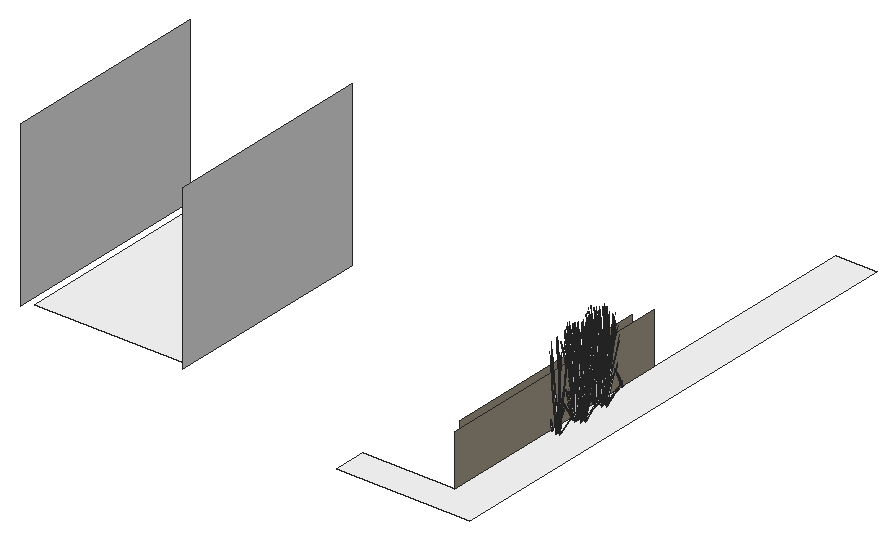
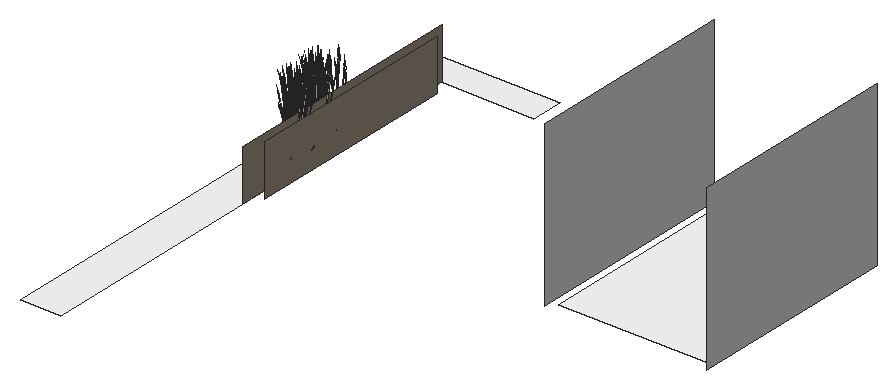
# SketchUp Ruby script. Lengths in inches.
U = 1.inch
M = Sketchup.active_model
def pt(a) = Geom::Point3d.new(a.map { |v| v * U })
def face(e, loops, mat)
  f = e.add_face(loops[0].map { |a| pt(a) })
  loops[1..].each { |l| e.add_face(l.map { |a| pt(a) }).erase! }
  f.material = f.back_material = mat if mat
  f
end
# faces: each face lists its corners as indices into pts; further lists are holes
def faces(e, pts, list, mat = nil) = list.each { |f| face(e, (f[0].is_a?(Array) ? f : [f]).map { |l| l.map { |i| pts[i] } }, mat) }
# xy, xz, yz: faces in a plane at the given z, y or x. An outline is a flat list of corners, or four numbers for a rectangle; further outlines are holes
def ring(l) = l.size == 4 ? [[l[0], l[1]], [l[2], l[1]], [l[2], l[3]], [l[0], l[3]]] : l.each_slice(2).to_a
def flat(e, list, mat, &to3) = list.each { |f| face(e, (f[0].is_a?(Array) ? f : [f]).map { |l| ring(l).map { |u, v| to3.(u, v) } }, mat) }
def xy(e, z, list, mat = nil) = flat(e, list, mat) { |x, y| [x, y, z] }
def xz(e, y, list, mat = nil) = flat(e, list, mat) { |x, z| [x, y, z] }
def yz(e, x, list, mat = nil) = flat(e, list, mat) { |y, z| [x, y, z] }
def lines(e, pts, list) = list.each { |a, b| e.add_line(pt(pts[a]), pt(pts[b])) }
# prism: a flat outline (further loops are holes) pulled along v
def prism(e, loops, v, mat = nil)
  f = face(e, loops, mat); d = Geom::Vector3d.new(v.map { |x| x * U })
  f.pushpull(f.normal.samedirection?(d) ? d.length : -d.length)
end
def box(e, o, s, mat = nil) = prism(e, [[o, [o[0] + s[0], o[1], o[2]], [o[0] + s[0], o[1] + s[1], o[2]], [o[0], o[1] + s[1], o[2]]]], [0, 0, s[2]], mat)
def at(x, y, z, deg = 0) = Geom::Transformation.translation(pt([x, y, z])) * Geom::Transformation.rotation(ORIGIN, Z_AXIS, deg.degrees)
def axes(o, x, y, z) = Geom::Transformation.new([*x, 0, *y, 0, *z, 0, *pt(o).to_a, 1])
def part(name) = M.definitions.add(name)
# library, detail: a bought-in or finely detailed component or shape, given as its bounding box
def library(name, o, s) = part(name).tap { |d| box(d.entities, o, s) }
def detail(e, o, s) = box(e.add_group.entities, o, s)
def put(e, d, t, mat = nil) = e.add_instance(d, t).tap { |i| i.material = mat if mat }
def group(e, t, mat = nil) = e.add_group.tap { |g| g.transformation = t; g.material = mat if mat }.entities
root = M.entities
M.materials.add("LightPink_Translucent").color = [144, 107, 117]
M.materials["LightPink_Translucent"].alpha = 0.75
M.materials.add("M00_Soft_Cloud").color = [255, 255, 255]
M.materials.add("Plaster_04_1K").color = [142, 132, 117]
M.materials.add("[Metal_Corrogated_Shiny]").color = [193, 193, 193]
c1 = part("blade")
p = [[2.15,0.21,22],[0,0.17,0],[0.09,0.45,0],[2.18,0.31,22],[2.29,0.31,22],[0.38,0.45,0],
  [2.48,0.24,33],[2.49,0.24,33],[2.48,0.22,33]]
faces(c1.entities,p,[[0,1,2,3],[4,5,2,3],[6,3,4,7],[8,0,3,6]])
c2 = part("seeds")
p = [[0.3,-0.1,1.38],[-0.01,-0.03,1.59],[-0.01,-0.03,0.03],[0.14,-0.07,-0.07],[0.29,-0.03,3],[0.15,0.01,3.11]]
faces(c2.entities,p,[[0,1,2,3],[1,0,4,5]],"LightPink_Translucent")
c3 = part("blade with seeds")
put(c3.entities,c1,at(0,0,0))
put(c3.entities,c2,axes([2.4,0.25,30.99],[1.5799,-0.05474,1.17369],[-0.12525,1.92788,0.29478],[-0.07173,-0.02425,1.56792]))
xy(root,255,[[333.82,39.98,432,39.98,432,414.98,402,414.98,402,63.98,333.82,63.98],[78,82.09,186,225.98]],"M00_Soft_Cloud")
yz(root,72,[[75.98,255,231.98,375]],"[Metal_Corrogated_Shiny]")
yz(root,192,[[75.98,255,231.98,375]],"[Metal_Corrogated_Shiny]")
yz(root,396,[[75.98,255,234.98,292.64]],"Plaster_04_1K")
yz(root,402,[[63.98,255,246.98,292.64]],"Plaster_04_1K")
put(root,c3,axes([409.78,148.04,257.21],[-0.36864,0.55059,-0.44739],[-0.76598,-0.26498,0.21531],[0,0.12692,1.43643]))
put(root,c3,axes([408.89,148.84,257.06],[-0.51177,0.45928,-0.62353],[-0.63575,-0.41646,-0.16365],[-0.20507,0.11457,1.37633]))
put(root,c3,axes([409.8,149.62,257.33],[0.95122,0.19861,0.30756],[-0.23797,0.7099,-0.36492],[-0.15744,0.08885,1.64885]))
put(root,c3,axes([409.73,150.1,257.02],[-0.7111,0.30552,-0.49651],[-0.42504,-0.54784,0],[-0.16196,0.06958,1.57504]))
put(root,c3,axes([412.09,148.29,257.02],[0,0.61104,-0.49651],[-0.85008,0,0],[0,0.13917,1.57504]))
put(root,c3,axes([410.375,150,257.375],[0.47504,0.61229,0],[-0.79476,0.34146,-0.51607],[-0.18101,0.07777,1.63711]))
put(root,c3,axes([411.13,150.21,256.49],[0.05536,-0.08822,1.76342],[0.69692,-0.25981,-0.26939],[0.21129,0.13447,0.30037]))
put(root,c3,axes([410.21,148.2,257.09],[0.2786,0.55945,-0.69212],[-0.80253,0.20149,-0.18165],[0.03079,0.18945,1.52773]))
put(root,c3,axes([404.73,150.13,256.49],[0.10192,0.06105,1.76342],[0.17281,0.56562,-0.26939],[-0.22588,0.12062,0.30037]))
put(root,c3,axes([407.875,150.1875,256.49],[0.12297,-0.03325,1.76342],[0.73967,0.18301,-0.26939],[0.02163,0.20626,0.30037]))
put(root,c3,axes([408.77,166.76,256.49],[-0.12744,0.02202,1.76342],[-0.70477,-0.24781,-0.26939],[0.01183,-0.2067,0.30037]))
put(root,c3,axes([406.49,167.52,256.49],[-0.0736,0.08049,1.76342],[-0.74378,0.17355,-0.26939],[-0.17968,-0.15788,0.30037]))
put(root,c3,axes([407.72,169.73,257.1],[-0.31203,-0.62659,-0.69835],[0.89884,-0.22566,-0.18329],[-0.03449,-0.21218,1.54149]))
put(root,c3,axes([411.89,167.82,256.49],[-0.11372,-0.04814,1.76342],[-0.29211,-0.53779,-0.26939],[0.19706,-0.14594,0.30037]))
put(root,c3,axes([407.6,167.93,257.375],[-0.47504,-0.61229,0],[0.79476,-0.34146,-0.51607],[0.18101,-0.07777,1.63711]))
put(root,c3,axes([408.64,167.19,257.13],[-0.52505,0.35054,-0.03893],[-0.48109,-0.38392,-0.17649],[-0.03387,-0.10878,0.58215]))
put(root,c3,axes([405.88,169.64,257.02],[0,-0.61104,-0.49651],[0.85008,0,0],[0,-0.13917,1.57504]))
put(root,c3,axes([408.24,167.84,257.02],[0.7111,-0.30552,-0.49651],[0.42504,0.54784,0],[0.16196,-0.06958,1.57504]))
put(root,c3,axes([409.08,169.09,257.06],[0.51177,-0.45928,-0.62353],[0.63575,0.41646,-0.16365],[0.20507,-0.11457,1.37633]))
put(root,c3,axes([408.19,169.89,257.21],[0.36864,-0.55059,-0.44739],[0.76598,0.26498,0.21531],[0,-0.12692,1.43643]))
put(root,c3,axes([408.53,169.62,257.67],[-0.08854,-0.69723,-0.29095],[0.92215,-0.04216,-0.50002],[0.16238,-0.09287,1.59708]))
put(root,c3,axes([406.24,169.66,257.03],[0.53038,-0.38124,-0.30978],[0.53038,0.38124,0.30978],[0,-0.1228,1.38974]))
put(root,c3,axes([406.03,167.83,257.13],[-0.21918,0.49894,-0.03893],[-0.6746,-0.15348,-0.17649],[-0.10242,-0.08161,0.58215]))
put(root,c3,axes([408.1,170.35,257.67],[-0.85568,-0.29155,-0.29095],[0.41201,-0.61537,-0.50002],[-0.02689,-0.15109,1.59708]))
put(root,c3,axes([405.67,170.11,257.375],[-0.95008,0,0],[0,-0.68292,-0.51607],[0,-0.15554,1.63711]))
put(root,c3,axes([408.41,168.08,257.03],[0.70886,0.15119,-0.30978],[-0.17848,0.53243,0.30978],[0.1429,-0.0614,1.38974]))
put(root,c3,axes([406.4,169.93,257.33],[-0.70674,0.51372,0.30756],[-0.70717,-0.50832,-0.36492],[-0.02468,-0.14589,1.64885]))
put(root,c3,axes([408.32,171,257.4375],[0.20138,-0.72405,-0.23429],[0.95485,0.12621,0.51271],[-0.16685,-0.09999,1.5644]))
put(root,c3,axes([411.09,168.08,257.375],[0.47504,-0.61229,0],[0.79476,0.34146,-0.51607],[0.18101,0.07777,1.63711]))
put(root,c3,axes([408.25,170.7,257.21],[-0.45644,-0.51287,-0.44739],[0.69137,-0.36116,0.21531],[-0.14771,-0.06346,1.43643]))
put(root,c3,axes([408.35,169.98,257.36],[0.33034,0.68327,0.45755],[-0.94388,0.2376,0.17955],[0.01154,-0.12555,1.58856]))
put(root,c3,axes([412.96,170.5,256.98],[-0.48937,0.07333,1.41583],[-0.07789,-0.58369,0.08104],[0.34275,-0.08835,0.80566]))
put(root,c3,axes([413.86,169.99,257.26],[-0.47106,-0.39072,-0.06488],[0.51591,-0.35801,-0.29416],[0.14618,-0.02521,0.97024]))
put(root,c3,axes([409.53,170.04,257.21],[0,-0.70701,0],[0.95008,0,0],[0,0,1.79456]))
put(root,c3,axes([407.84,170.9,257.06],[-0.79037,-0.10018,-0.62353],[0.16679,-0.61794,-0.16365],[-0.23587,-0.07488,1.37633]))
put(root,c3,axes([409.08,169.59,257.36],[-0.62999,0.55453,0.45755],[-0.74845,-0.4895,0.17955],[0.15188,-0.05534,1.58856]))
put(root,c3,axes([409.77,170.59,257.3],[-0.70674,-0.52593,-0.06131],[0.70717,-0.52625,0],[-0.02468,-0.01837,1.75571]))
put(root,c3,axes([407.66,169.17,256.59],[-0.74787,0.24464,1.28929],[-0.23804,-0.70192,0.50096],[0.45924,0.01168,1.46642]))
put(root,c3,axes([408.43,170.65,257.36],[0.96033,0.12874,0.45755],[-0.19544,0.7271,0.17955],[-0.14034,-0.07021,1.58856]))
put(root,c3,axes([413.5,170.125,256.49],[-0.03971,-0.09277,1.76342],[0.27541,-0.54264,-0.26939],[0.27782,-0.00781,0.30037]))
put(root,c3,axes([405.3,170.03,256.49],[0.01927,0.0963,1.76342],[-0.38846,0.5029,-0.26939],[-0.27592,-0.02535,0.30037]))
put(root,c3,axes([407,171.84,257.03],[-0.17848,-0.53243,-0.30978],[0.70886,-0.15119,0.30978],[-0.1429,-0.0614,1.38974]))
put(root,c3,axes([409.59,169.53,257.67],[0.76714,-0.40567,-0.29095],[0.51013,0.57321,-0.50002],[0.18927,0.05821,1.59708]))
put(root,c3,axes([406.8,172.07,257.02],[-0.7111,-0.30552,-0.49651],[0.42504,-0.54784,0],[-0.16196,-0.06958,1.57504]))
put(root,c3,axes([411.53,168.45,257.02],[0.7111,0.30552,-0.49651],[-0.42504,0.54784,0],[0.16196,0.06958,1.57504]))
put(root,c3,axes([410.18,170.2,257.21],[0.85008,0,0],[0,0.63259,0],[0,0,1.78407]))
put(root,c3,axes([408.74,170.99,257.67],[-0.76714,0.40567,-0.29095],[-0.51013,-0.57321,-0.50002],[-0.18927,-0.05821,1.59708]))
put(root,c3,axes([411.33,168.68,257.03],[0.17848,0.53243,-0.30978],[-0.70886,0.15119,0.30978],[0.1429,0.0614,1.38974]))
put(root,c3,axes([409.14,171.67,257.2],[-0.24791,-0.5268,0],[0.70791,-0.18448,0],[0,0,1.54371]))
put(root,c3,axes([410.07,171.6,257.18],[0.79769,-0.20732,-0.19198],[0.2803,0.59721,0.00008],[0.08805,-0.02292,1.73897]))
put(root,c3,axes([410.16,170.47,257.21],[0.53038,0.39469,0],[-0.53038,0.39469,0],[0,0,1.69266]))
put(root,c3,axes([410.49,169.625,257.06],[0.79037,0.10018,-0.62353],[-0.16679,0.61794,-0.16365],[0.23587,0.07488,1.37633]))
put(root,c3,axes([408.96,171.91,257.2],[-0.76598,-0.27433,0],[0.36864,-0.57001,0],[0,0,1.62707]))
put(root,c3,axes([409.6,171.18,257.46],[-0.74193,-0.49181,-0.25192],[0.6243,-0.55226,0.5513],[-0.19979,0.05753,1.68216]))
put(root,c3,axes([410.01,170.32,257.29],[0,0.70667,-0.05637],[-0.95008,0,0],[0,0.02221,1.79368]))
put(root,c3,axes([410.08,169.82,257.21],[0.45644,0.51287,-0.44739],[-0.69137,0.36116,0.21531],[0.14771,0.06346,1.43643]))
put(root,c3,axes([407.24,172.44,257.375],[-0.47504,0.61229,0],[-0.79476,-0.34146,-0.51607],[-0.18101,-0.07777,1.63711]))
put(root,c3,axes([409.22,171.07,257.21],[-0.82508,0.03772,-0.44739],[-0.07462,-0.62614,0.21531],[-0.14771,0.06346,1.43643]))
put(root,c3,axes([409.83,171.92,257.2],[0.76598,0.27433,0],[-0.36864,0.57001,0],[0,0,1.74954]))
put(root,c3,axes([410.14,172.53,257.19],[-0.46912,-0.61443,-0.05142],[0.79476,-0.34146,0.51607],[-0.19584,0.0585,1.6363]))
put(root,c3,axes([409.56,171.6875,257.29],[0.33034,0.70197,-0.06012],[-0.94388,0.24598,0],[0.01154,0.02451,1.72173]))
put(root,c3,axes([409.92,172.45,257.03],[-0.70886,-0.15119,-0.30978],[0.17848,-0.53243,0.30978],[-0.1429,0.0614,1.38974]))
put(root,c3,axes([412.66,170.42,257.375],[0.95008,0,0],[0,0.68292,-0.51607],[0,0.15554,1.63711]))
put(root,c3,axes([412.29,170.77,257.2],[-0.94962,-0.00489,-0.04976],[0,-0.68292,0.49943],[-0.02984,0.15546,1.58352]))
put(root,c3,axes([410.23,170.17,257.67],[0.85568,0.29155,-0.29095],[-0.41201,0.61537,-0.50002],[0.02689,0.15109,1.59708]))
put(root,c3,axes([412.09,170.87,257.03],[-0.53038,0.38124,-0.30978],[-0.53038,-0.38124,0.30978],[0,0.1228,1.38974]))
put(root,c3,axes([409.8,170.9,257.67],[0.08854,0.69723,-0.29095],[-0.92215,0.04216,-0.50002],[-0.16238,0.09287,1.59708]))
put(root,c3,axes([410.14,170.63,257.21],[-0.36864,0.55059,-0.44739],[-0.76598,-0.26498,0.21531],[0,0.12692,1.43643]))
put(root,c3,axes([409.25,171.4375,257.06],[-0.51177,0.45928,-0.62353],[-0.63575,-0.41646,-0.16365],[-0.20507,0.11457,1.37633]))
put(root,c3,axes([410.16,172.21,257.33],[0.95122,0.19861,0.30756],[-0.23797,0.7099,-0.36492],[-0.15744,0.08885,1.64885]))
put(root,c3,axes([410.09,172.6875,257.02],[-0.7111,0.30552,-0.49651],[-0.42504,-0.54784,0],[-0.16196,0.06958,1.57504]))
put(root,c3,axes([412.45,170.88,257.02],[0,0.61104,-0.49651],[-0.85008,0,0],[0,0.13917,1.57504]))
put(root,c3,axes([410.74,172.59,257.375],[0.47504,0.61229,0],[-0.79476,0.34146,-0.51607],[-0.18101,0.07777,1.63711]))
put(root,c3,axes([411.49,172.8,256.49],[0.05536,-0.08822,1.76342],[0.69692,-0.25981,-0.26939],[0.21129,0.13447,0.30037]))
put(root,c3,axes([410.57,170.8,257.09],[0.2786,0.55945,-0.69212],[-0.80253,0.20149,-0.18165],[0.03079,0.18945,1.52773]))
put(root,c3,axes([405.09,172.73,256.49],[0.10192,0.06105,1.76342],[0.17281,0.56562,-0.26939],[-0.22588,0.12062,0.30037]))
put(root,c3,axes([408.24,172.78,256.49],[0.12297,-0.03325,1.76342],[0.73967,0.18301,-0.26939],[0.02163,0.20626,0.30037]))
put(root,c3,axes([406.75,188.89,256.49],[-0.12744,0.02202,1.76342],[-0.70477,-0.24781,-0.26939],[0.01183,-0.2067,0.30037]))
put(root,c3,axes([404.47,189.65,256.49],[-0.0736,0.08049,1.76342],[-0.74378,0.17355,-0.26939],[-0.17968,-0.15788,0.30037]))
put(root,c3,axes([405.7,191.86,257.1],[-0.31203,-0.62659,-0.69835],[0.89884,-0.22566,-0.18329],[-0.03449,-0.21218,1.54149]))
put(root,c3,axes([409.87,189.95,256.49],[-0.11372,-0.04814,1.76342],[-0.29211,-0.53779,-0.26939],[0.19706,-0.14594,0.30037]))
put(root,c3,axes([405.58,190.0625,257.375],[-0.47504,-0.61229,0],[0.79476,-0.34146,-0.51607],[0.18101,-0.07777,1.63711]))
put(root,c3,axes([406.62,189.32,257.13],[-0.52505,0.35054,-0.03893],[-0.48109,-0.38392,-0.17649],[-0.03387,-0.10878,0.58215]))
put(root,c3,axes([403.86,191.78,257.02],[0,-0.61104,-0.49651],[0.85008,0,0],[0,-0.13917,1.57504]))
put(root,c3,axes([406.22,189.97,257.02],[0.7111,-0.30552,-0.49651],[0.42504,0.54784,0],[0.16196,-0.06958,1.57504]))
put(root,c3,axes([407.07,191.22,257.06],[0.51177,-0.45928,-0.62353],[0.63575,0.41646,-0.16365],[0.20507,-0.11457,1.37633]))
put(root,c3,axes([406.17,192.02,257.21],[0.36864,-0.55059,-0.44739],[0.76598,0.26498,0.21531],[0,-0.12692,1.43643]))
put(root,c3,axes([406.51,191.75,257.67],[-0.08854,-0.69723,-0.29095],[0.92215,-0.04216,-0.50002],[0.16238,-0.09287,1.59708]))
put(root,c3,axes([404.23,191.79,257.03],[0.53038,-0.38124,-0.30978],[0.53038,0.38124,0.30978],[0,-0.1228,1.38974]))
put(root,c3,axes([404.01,189.96,257.13],[-0.21918,0.49894,-0.03893],[-0.6746,-0.15348,-0.17649],[-0.10242,-0.08161,0.58215]))
put(root,c3,axes([406.08,192.48,257.67],[-0.85568,-0.29155,-0.29095],[0.41201,-0.61537,-0.50002],[-0.02689,-0.15109,1.59708]))
put(root,c3,axes([403.65,192.24,257.375],[-0.95008,0,0],[0,-0.68292,-0.51607],[0,-0.15554,1.63711]))
put(root,c3,axes([406.39,190.21,257.03],[0.70886,0.15119,-0.30978],[-0.17848,0.53243,0.30978],[0.1429,-0.0614,1.38974]))
put(root,c3,axes([404.38,192.06,257.33],[-0.70674,0.51372,0.30756],[-0.70717,-0.50832,-0.36492],[-0.02468,-0.14589,1.64885]))
put(root,c3,axes([406.3,193.13,257.4375],[0.20138,-0.72405,-0.23429],[0.95485,0.12621,0.51271],[-0.16685,-0.09999,1.5644]))
put(root,c3,axes([409.08,190.22,257.375],[0.47504,-0.61229,0],[0.79476,0.34146,-0.51607],[0.18101,0.07777,1.63711]))
put(root,c3,axes([406.23,192.84,257.21],[-0.45644,-0.51287,-0.44739],[0.69137,-0.36116,0.21531],[-0.14771,-0.06346,1.43643]))
put(root,c3,axes([406.33,192.11,257.36],[0.33034,0.68327,0.45755],[-0.94388,0.2376,0.17955],[0.01154,-0.12555,1.58856]))
put(root,c3,axes([410.95,192.64,256.98],[-0.48937,0.07333,1.41583],[-0.07789,-0.58369,0.08104],[0.34275,-0.08835,0.80566]))
put(root,c3,axes([411.84,192.12,257.26],[-0.47106,-0.39072,-0.06488],[0.51591,-0.35801,-0.29416],[0.14618,-0.02521,0.97024]))
put(root,c3,axes([407.51,192.17,257.21],[0,-0.70701,0],[0.95008,0,0],[0,0,1.79456]))
put(root,c3,axes([405.82,193.03,257.06],[-0.79037,-0.10018,-0.62353],[0.16679,-0.61794,-0.16365],[-0.23587,-0.07488,1.37633]))
put(root,c3,axes([407.06,191.72,257.36],[-0.62999,0.55453,0.45755],[-0.74845,-0.4895,0.17955],[0.15188,-0.05534,1.58856]))
put(root,c3,axes([407.75,192.72,257.3],[-0.70674,-0.52593,-0.06131],[0.70717,-0.52625,0],[-0.02468,-0.01837,1.75571]))
put(root,c3,axes([405.64,191.3,256.59],[-0.74787,0.24464,1.28929],[-0.23804,-0.70192,0.50096],[0.45924,0.01168,1.46642]))
put(root,c3,axes([406.41,192.78,257.36],[0.96033,0.12874,0.45755],[-0.19544,0.7271,0.17955],[-0.14034,-0.07021,1.58856]))
put(root,c3,axes([411.48,192.25,256.49],[-0.03971,-0.09277,1.76342],[0.27541,-0.54264,-0.26939],[0.27782,-0.00781,0.30037]))
put(root,c3,axes([403.28,192.16,256.49],[0.01927,0.0963,1.76342],[-0.38846,0.5029,-0.26939],[-0.27592,-0.02535,0.30037]))
put(root,c3,axes([404.98,193.97,257.03],[-0.17848,-0.53243,-0.30978],[0.70886,-0.15119,0.30978],[-0.1429,-0.0614,1.38974]))
put(root,c3,axes([407.58,191.66,257.67],[0.76714,-0.40567,-0.29095],[0.51013,0.57321,-0.50002],[0.18927,0.05821,1.59708]))
put(root,c3,axes([404.79,194.2,257.02],[-0.7111,-0.30552,-0.49651],[0.42504,-0.54784,0],[-0.16196,-0.06958,1.57504]))
put(root,c3,axes([409.51,190.58,257.02],[0.7111,0.30552,-0.49651],[-0.42504,0.54784,0],[0.16196,0.06958,1.57504]))
put(root,c3,axes([408.16,192.33,257.21],[0.85008,0,0],[0,0.63259,0],[0,0,1.78407]))
put(root,c3,axes([406.72,193.125,257.67],[-0.76714,0.40567,-0.29095],[-0.51013,-0.57321,-0.50002],[-0.18927,-0.05821,1.59708]))
put(root,c3,axes([409.3125,190.8125,257.03],[0.17848,0.53243,-0.30978],[-0.70886,0.15119,0.30978],[0.1429,0.0614,1.38974]))
put(root,c3,axes([407.12,193.8,257.2],[-0.24791,-0.5268,0],[0.70791,-0.18448,0],[0,0,1.54371]))
put(root,c3,axes([408.05,193.73,257.18],[0.79769,-0.20732,-0.19198],[0.2803,0.59721,0.00008],[0.08805,-0.02292,1.73897]))
put(root,c3,axes([408.14,192.6,257.21],[0.53038,0.39469,0],[-0.53038,0.39469,0],[0,0,1.69266]))
put(root,c3,axes([408.47,191.75,257.06],[0.79037,0.10018,-0.62353],[-0.16679,0.61794,-0.16365],[0.23587,0.07488,1.37633]))
put(root,c3,axes([406.94,194.04,257.2],[-0.76598,-0.27433,0],[0.36864,-0.57001,0],[0,0,1.62707]))
put(root,c3,axes([407.58,193.31,257.46],[-0.74193,-0.49181,-0.25192],[0.6243,-0.55226,0.5513],[-0.19979,0.05753,1.68216]))
put(root,c3,axes([407.99,192.45,257.29],[0,0.70667,-0.05637],[-0.95008,0,0],[0,0.02221,1.79368]))
put(root,c3,axes([408.0625,191.95,257.21],[0.45644,0.51287,-0.44739],[-0.69137,0.36116,0.21531],[0.14771,0.06346,1.43643]))
put(root,c3,axes([405.22,194.57,257.375],[-0.47504,0.61229,0],[-0.79476,-0.34146,-0.51607],[-0.18101,-0.07777,1.63711]))
put(root,c3,axes([407.2,193.2,257.21],[-0.82508,0.03772,-0.44739],[-0.07462,-0.62614,0.21531],[-0.14771,0.06346,1.43643]))
put(root,c3,axes([407.8125,194.05,257.2],[0.76598,0.27433,0],[-0.36864,0.57001,0],[0,0,1.74954]))
put(root,c3,axes([408.12,194.66,257.19],[-0.46912,-0.61443,-0.05142],[0.79476,-0.34146,0.51607],[-0.19584,0.0585,1.6363]))
put(root,c3,axes([407.54,193.82,257.29],[0.33034,0.70197,-0.06012],[-0.94388,0.24598,0],[0.01154,0.02451,1.72173]))
put(root,c3,axes([407.9,194.58,257.03],[-0.70886,-0.15119,-0.30978],[0.17848,-0.53243,0.30978],[-0.1429,0.0614,1.38974]))
put(root,c3,axes([410.65,192.55,257.375],[0.95008,0,0],[0,0.68292,-0.51607],[0,0.15554,1.63711]))
put(root,c3,axes([410.27,192.9,257.2],[-0.94962,-0.00489,-0.04976],[0,-0.68292,0.49943],[-0.02984,0.15546,1.58352]))
put(root,c3,axes([408.21,192.3,257.67],[0.85568,0.29155,-0.29095],[-0.41201,0.61537,-0.50002],[0.02689,0.15109,1.59708]))
put(root,c3,axes([410.07,193,257.03],[-0.53038,0.38124,-0.30978],[-0.53038,-0.38124,0.30978],[0,0.1228,1.38974]))
put(root,c3,axes([407.78,193.03,257.67],[0.08854,0.69723,-0.29095],[-0.92215,0.04216,-0.50002],[-0.16238,0.09287,1.59708]))
put(root,c3,axes([408.12,192.76,257.21],[-0.36864,0.55059,-0.44739],[-0.76598,-0.26498,0.21531],[0,0.12692,1.43643]))
put(root,c3,axes([407.23,193.57,257.06],[-0.51177,0.45928,-0.62353],[-0.63575,-0.41646,-0.16365],[-0.20507,0.11457,1.37633]))
put(root,c3,axes([408.14,194.34,257.33],[0.95122,0.19861,0.30756],[-0.23797,0.7099,-0.36492],[-0.15744,0.08885,1.64885]))
put(root,c3,axes([408.07,194.82,257.02],[-0.7111,0.30552,-0.49651],[-0.42504,-0.54784,0],[-0.16196,0.06958,1.57504]))
put(root,c3,axes([410.43,193.01,257.02],[0,0.61104,-0.49651],[-0.85008,0,0],[0,0.13917,1.57504]))
put(root,c3,axes([408.72,194.73,257.375],[0.47504,0.61229,0],[-0.79476,0.34146,-0.51607],[-0.18101,0.07777,1.63711]))
put(root,c3,axes([409.47,194.93,256.49],[0.05536,-0.08822,1.76342],[0.69692,-0.25981,-0.26939],[0.21129,0.13447,0.30037]))
put(root,c3,axes([408.55,192.93,257.09],[0.2786,0.55945,-0.69212],[-0.80253,0.20149,-0.18165],[0.03079,0.18945,1.52773]))
put(root,c3,axes([403.07,194.86,256.49],[0.10192,0.06105,1.76342],[0.17281,0.56562,-0.26939],[-0.22588,0.12062,0.30037]))
put(root,c3,axes([406.22,194.91,256.49],[0.12297,-0.03325,1.76342],[0.73967,0.18301,-0.26939],[0.02163,0.20626,0.30037]))
put(root,c3,axes([404.35,215.65,256.49],[-0.12744,0.02202,1.76342],[-0.70477,-0.24781,-0.26939],[0.01183,-0.2067,0.30037]))
put(root,c3,axes([402.07,216.41,256.49],[-0.0736,0.08049,1.76342],[-0.74378,0.17355,-0.26939],[-0.17968,-0.15788,0.30037]))
